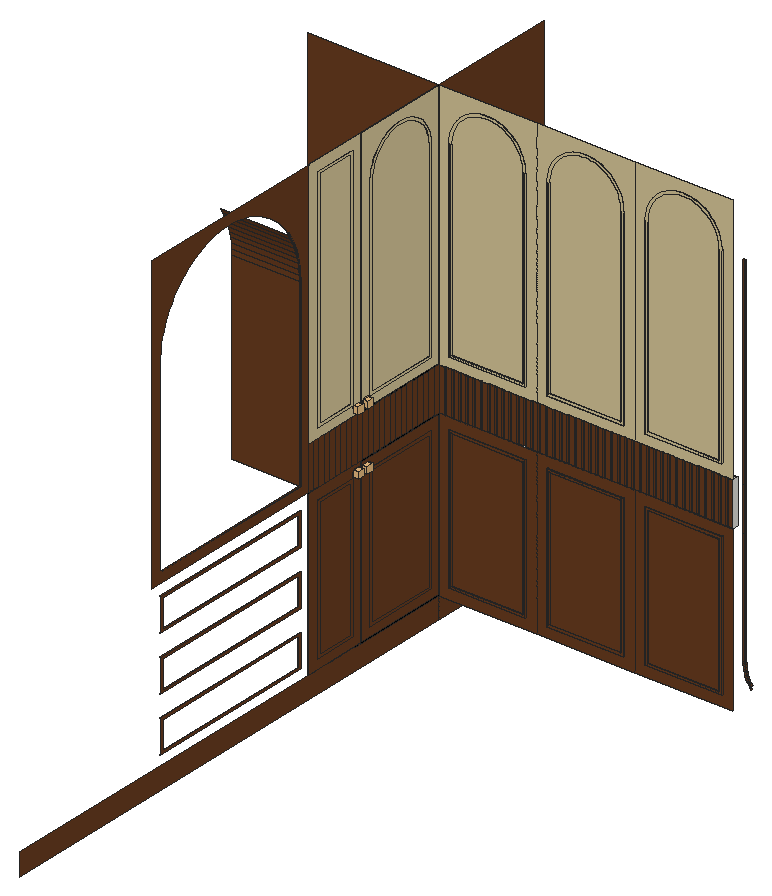
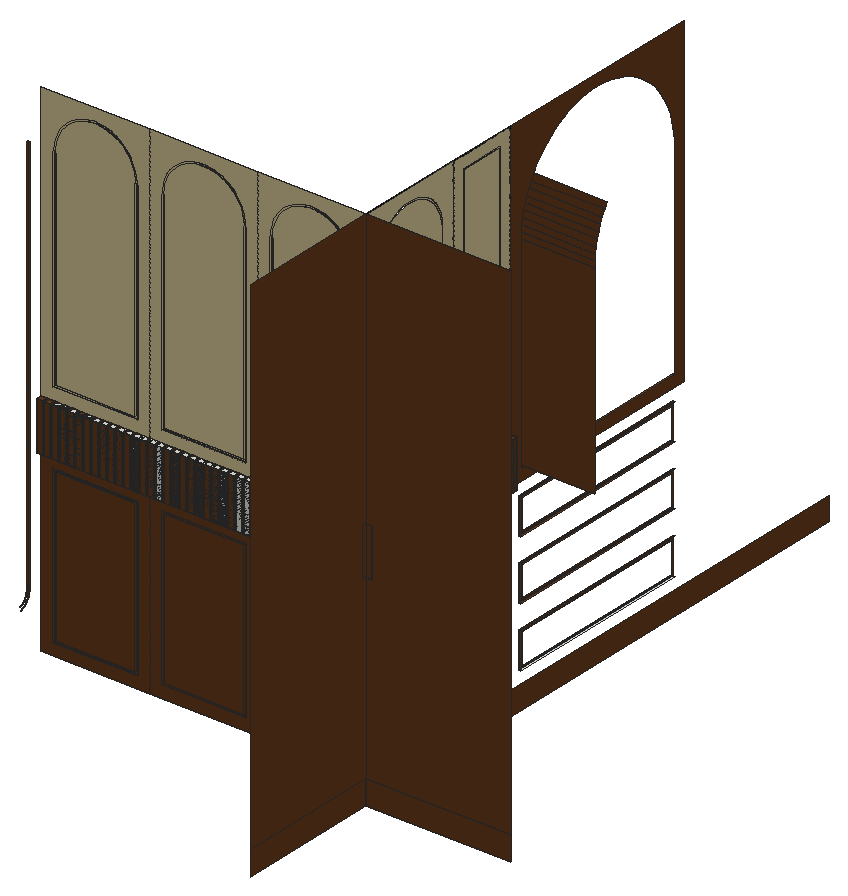
# SketchUp Ruby script. Lengths in inches.
U = 1.inch
M = Sketchup.active_model
def pt(a) = Geom::Point3d.new(a.map { |v| v * U })
def face(e, loops, mat)
  f = e.add_face(loops[0].map { |a| pt(a) })
  loops[1..].each { |l| e.add_face(l.map { |a| pt(a) }).erase! }
  f.material = f.back_material = mat if mat
  f
end
# faces: each face lists its corners as indices into pts; further lists are holes
def faces(e, pts, list, mat = nil) = list.each { |f| face(e, (f[0].is_a?(Array) ? f : [f]).map { |l| l.map { |i| pts[i] } }, mat) }
# xy, xz, yz: faces in a plane at the given z, y or x. An outline is a flat list of corners, or four numbers for a rectangle; further outlines are holes
def ring(l) = l.size == 4 ? [[l[0], l[1]], [l[2], l[1]], [l[2], l[3]], [l[0], l[3]]] : l.each_slice(2).to_a
def flat(e, list, mat, &to3) = list.each { |f| face(e, (f[0].is_a?(Array) ? f : [f]).map { |l| ring(l).map { |u, v| to3.(u, v) } }, mat) }
def xy(e, z, list, mat = nil) = flat(e, list, mat) { |x, y| [x, y, z] }
def xz(e, y, list, mat = nil) = flat(e, list, mat) { |x, z| [x, y, z] }
def yz(e, x, list, mat = nil) = flat(e, list, mat) { |y, z| [x, y, z] }
def lines(e, pts, list) = list.each { |a, b| e.add_line(pt(pts[a]), pt(pts[b])) }
# prism: a flat outline (further loops are holes) pulled along v
def prism(e, loops, v, mat = nil)
  f = face(e, loops, mat); d = Geom::Vector3d.new(v.map { |x| x * U })
  f.pushpull(f.normal.samedirection?(d) ? d.length : -d.length)
end
def box(e, o, s, mat = nil) = prism(e, [[o, [o[0] + s[0], o[1], o[2]], [o[0] + s[0], o[1] + s[1], o[2]], [o[0], o[1] + s[1], o[2]]]], [0, 0, s[2]], mat)
def at(x, y, z, deg = 0) = Geom::Transformation.translation(pt([x, y, z])) * Geom::Transformation.rotation(ORIGIN, Z_AXIS, deg.degrees)
def axes(o, x, y, z) = Geom::Transformation.new([*x, 0, *y, 0, *z, 0, *pt(o).to_a, 1])
def part(name) = M.definitions.add(name)
# library, detail: a bought-in or finely detailed component or shape, given as its bounding box
def library(name, o, s) = part(name).tap { |d| box(d.entities, o, s) }
def detail(e, o, s) = box(e.add_group.entities, o, s)
def put(e, d, t, mat = nil) = e.add_instance(d, t).tap { |i| i.material = mat if mat }
def group(e, t, mat = nil) = e.add_group.tap { |g| g.transformation = t; g.material = mat if mat }.entities
root = M.entities
M.materials.add("138_plaster painted wall texture-seamless").color = [214, 198, 153]
M.materials.add("[0137_Black]").color = [0, 0, 0]
M.materials.add("[Wood Veneer 01]").color = [104, 60, 32]
c1 = part("Group\#7")
box(c1.entities,[0,0,0],[1,1,8])
c2 = library("Group\#17",[0,0,0],[1.625,1.625,1.31])
c3 = part("Square post")
box(c3.entities,[0,0,0],[1,1,8])
xy(root,6,[[24,56,24.2,88],[24,92,24.2,100],[24,104,24.2,118],[26,119.8,40,120],[44,119.8,58,120]])
xy(root,6,[[62,119.8,76,120]],"[Wood Veneer 01]")
xy(root,6.4,[[24,56.4,24.2,87.6],[24,92.4,24.2,99.6],[24,104.4,24.2,117.6],[26.4,119.8,39.6,120],[44.4,119.8,57.6,120],
  [62.4,119.8,75.6,120]],"[Wood Veneer 01]")
xy(root,11.6,[[24,56.4,24.2,87.6]])
xy(root,12,[[24,56,24.2,88]],"[Wood Veneer 01]")
xy(root,16,[[24,56,24.2,88]],"[Wood Veneer 01]")
xy(root,16.4,[[24,56.4,24.2,87.6]],"[Wood Veneer 01]")
xy(root,21.6,[[24,56.4,24.2,87.6]],"[Wood Veneer 01]")
xy(root,22,[[24,56,24.2,88]],"[Wood Veneer 01]")
xy(root,26,[[24,56,24.2,88]],"[Wood Veneer 01]")
xy(root,26.4,[[24,56.4,24.2,87.6]],"[Wood Veneer 01]")
xy(root,31.6,[[24,56.4,24.2,87.6],[24,92.4,24.2,99.6],[24,104.4,24.2,117.6],[26.4,119.8,39.6,120],[44.4,119.8,57.6,120],
  [62.4,119.8,75.6,120]],"[Wood Veneer 01]")
xy(root,32,[[24,56,24.2,88],[24,92,24.2,100],[24,104,24.2,118],[26,119.8,40,120],[44,119.8,58,120],
  [62,119.8,76,120]],"[Wood Veneer 01]")
xy(root,34,[[24,120,42,121],[42,120,60,121],[60,120,78,121]])
xy(root,34,[[23,90,24,102],[23,102,24,120]],"[Wood Veneer 01]")
xy(root,36,[[24,56,24.2,88]],"[Wood Veneer 01]")
xy(root,42,[[24,120,42,121],[42,120,60,121],[60,120,78,121]])
xy(root,42,[[23,90,24,102],[23,102,24,120]],"[Wood Veneer 01]")
xy(root,44,[[24,92,24.2,100],[24,104,24.2,118],[26,119.8,40,120],[44,119.8,58,120],[62,119.8,76,120]])
xy(root,44.4,[[24,92.4,24.2,99.6],[24,104.4,24.2,117.6]])
xy(root,44.4,[[26.4,119.8,39.6,120],[44.4,119.8,57.6,120],[62.4,119.8,75.6,120]],"138_plaster painted wall texture-seamless")
xz(root,87.6,[[24,6.4,24.2,11.6],[24,16.4,24.2,21.6],[24,26.4,24.2,31.6],[12,36.4,24.2,70]],"[Wood Veneer 01]")
xz(root,88,[[24,6,24.2,12],[24,16,24.2,22],[24,26,24.2,32],[24,36,24.2,42],[24,42,24.2,70]],"[Wood Veneer 01]")
xz(root,90,[[23,34,24,42]])
xz(root,92,[[24,44,24.2,86]])
xz(root,92,[[24,6,24.2,32]],"[Wood Veneer 01]")
xz(root,92.4,[[24,44.4,24.2,85.6]])
xz(root,92.4,[[24,6.4,24.2,31.6]],"[Wood Veneer 01]")
xz(root,99.6,[[24,44.4,24.2,85.6]])
xz(root,99.6,[[24,6.4,24.2,31.6]],"[Wood Veneer 01]")
xz(root,100,[[24,44,24.2,86]])
xz(root,100,[[24,6,24.2,32]],"[Wood Veneer 01]")
xz(root,104,[[24,44,24.2,79]])
xz(root,104,[[24,6,24.2,32]],"[Wood Veneer 01]")
xz(root,104.4,[[24,44.4,24.2,79]])
xz(root,104.4,[[24,6.4,24.2,31.6]],"[Wood Veneer 01]")
xz(root,117.6,[[24,44.4,24.2,79]])
xz(root,117.6,[[24,6.4,24.2,31.6]],"[Wood Veneer 01]")
xz(root,118,[[24,44,24.2,79]])
xz(root,118,[[24,6,24.2,32]],"[Wood Veneer 01]")
xz(root,119.8,[[[26,44,40,44,40,79,39.99,79.46,39.94,79.91,39.87,80.37,39.76,80.8125,39.63,81.25,39.47,81.68,39.28,82.1,39.0625,82.5,38.82,82.89,38.55,83.26,38.26,83.62,37.95,83.95,37.62,84.26,37.26,84.55,36.89,84.82,36.5,85.0625,36.1,85.28,35.68,85.47,35.25,85.63,34.8125,85.76,34.37,85.87,33.91,85.94,33.46,85.99,33,86,32.54,85.99,32.09,85.94,31.63,85.87,31.1875,85.76,30.75,85.63,30.32,85.47,29.9,85.28,29.5,85.0625,29.11,84.82,28.74,84.55,28.38,84.26,28.05,83.95,27.74,83.62,27.45,83.26,27.18,82.89,26.9375,82.5,26.72,82.1,26.53,81.68,26.37,81.25,26.24,80.8125,26.13,80.37,26.06,79.91,26.01,79.46,26,79],[26.4,44.4,26.4,79,26.41,79.43,26.46,79.86,26.53,80.29,26.625,80.71,26.75,81.12,26.9,81.53,27.08,81.92,27.28,82.3,27.51,82.67,27.76,83.02,28.04,83.35,28.33,83.67,28.65,83.96,28.98,84.24,29.33,84.49,29.7,84.72,30.08,84.92,30.47,85.1,30.88,85.25,31.29,85.375,31.71,85.47,32.14,85.54,32.57,85.59,33,85.6,33.43,85.59,33.86,85.54,34.29,85.47,34.71,85.375,35.12,85.25,35.53,85.1,35.92,84.92,36.3,84.72,36.67,84.49,37.02,84.24,37.35,83.96,37.67,83.67,37.96,83.35,38.24,83.02,38.49,82.67,38.72,82.3,38.92,81.92,39.1,81.53,39.25,81.12,39.375,80.71,39.47,80.29,39.54,79.86,39.59,79.43,39.6,79,39.6,44.4]],[[44,44,58,44,58,79,57.99,79.46,57.94,79.91,57.87,80.37,57.76,80.8125,57.63,81.25,57.47,81.68,57.28,82.1,57.0625,82.5,56.82,82.89,56.55,83.26,56.26,83.62,55.95,83.95,55.62,84.26,55.26,84.55,54.89,84.82,54.5,85.0625,54.1,85.28,53.68,85.47,53.25,85.63,52.8125,85.76,52.37,85.87,51.91,85.94,51.46,85.99,51,86,50.54,85.99,50.09,85.94,49.63,85.87,49.1875,85.76,48.75,85.63,48.32,85.47,47.9,85.28,47.5,85.0625,47.11,84.82,46.74,84.55,46.38,84.26,46.05,83.95,45.74,83.62,45.45,83.26,45.18,82.89,44.9375,82.5,44.72,82.1,44.53,81.68,44.37,81.25,44.24,80.8125,44.13,80.37,44.06,79.91,44.01,79.46,44,79],[44.4,44.4,44.4,79,44.41,79.43,44.46,79.86,44.53,80.29,44.625,80.71,44.75,81.12,44.9,81.53,45.08,81.92,45.28,82.3,45.51,82.67,45.76,83.02,46.04,83.35,46.33,83.67,46.65,83.96,46.98,84.24,47.33,84.49,47.7,84.72,48.08,84.92,48.47,85.1,48.88,85.25,49.29,85.375,49.71,85.47,50.14,85.54,50.57,85.59,51,85.6,51.43,85.59,51.86,85.54,52.29,85.47,52.71,85.375,53.12,85.25,53.53,85.1,53.92,84.92,54.3,84.72,54.67,84.49,55.02,84.24,55.35,83.96,55.67,83.67,55.96,83.35,56.24,83.02,56.49,82.67,56.72,82.3,56.92,81.92,57.1,81.53,57.25,81.12,57.375,80.71,57.47,80.29,57.54,79.86,57.59,79.43,57.6,79,57.6,44.4]],[[62,44,76,44,76,79,75.99,79.46,75.94,79.91,75.87,80.37,75.76,80.8125,75.63,81.25,75.47,81.68,75.28,82.1,75.0625,82.5,74.82,82.89,74.55,83.26,74.26,83.62,73.95,83.95,73.62,84.26,73.26,84.55,72.89,84.82,72.5,85.0625,72.1,85.28,71.68,85.47,71.25,85.63,70.8125,85.76,70.37,85.87,69.91,85.94,69.46,85.99,69,86,68.54,85.99,68.09,85.94,67.63,85.87,67.1875,85.76,66.75,85.63,66.32,85.47,65.9,85.28,65.5,85.0625,65.11,84.82,64.74,84.55,64.38,84.26,64.05,83.95,63.74,83.62,63.45,83.26,63.18,82.89,62.9375,82.5,62.72,82.1,62.53,81.68,62.37,81.25,62.24,80.8125,62.13,80.37,62.06,79.91,62.01,79.46,62,79],[62.4,44.4,62.4,79,62.41,79.43,62.46,79.86,62.53,80.29,62.625,80.71,62.75,81.12,62.9,81.53,63.08,81.92,63.28,82.3,63.51,82.67,63.76,83.02,64.04,83.35,64.33,83.67,64.65,83.96,64.98,84.24,65.33,84.49,65.7,84.72,66.08,84.92,66.47,85.1,66.88,85.25,67.29,85.375,67.71,85.47,68.14,85.54,68.57,85.59,69,85.6,69.43,85.59,69.86,85.54,70.29,85.47,70.71,85.375,71.12,85.25,71.53,85.1,71.92,84.92,72.3,84.72,72.67,84.49,73.02,84.24,73.35,83.96,73.67,83.67,73.96,83.35,74.24,83.02,74.49,82.67,74.72,82.3,74.92,81.92,75.1,81.53,75.25,81.12,75.375,80.71,75.47,80.29,75.54,79.86,75.59,79.43,75.6,79,75.6,44.4]]],"138_plaster painted wall texture-seamless")
xz(root,119.8,[[[26,6,40,32],[26.4,6.4,39.6,31.6]],[[44,6,58,32],[44.4,6.4,57.6,31.6]],[[62,6,76,32],[62.4,6.4,75.6,31.6]]],"[Wood Veneer 01]")
xz(root,120,[[[24,42,42,88],[26,44,26,79,26.01,79.46,26.06,79.91,26.13,80.37,26.24,80.8125,26.37,81.25,26.53,81.68,26.72,82.1,26.9375,82.5,27.18,82.89,27.45,83.26,27.74,83.62,28.05,83.95,28.38,84.26,28.74,84.55,29.11,84.82,29.5,85.0625,29.9,85.28,30.32,85.47,30.75,85.63,31.1875,85.76,31.63,85.87,32.09,85.94,32.54,85.99,33,86,33.46,85.99,33.91,85.94,34.37,85.87,34.8125,85.76,35.25,85.63,35.68,85.47,36.1,85.28,36.5,85.0625,36.89,84.82,37.26,84.55,37.62,84.26,37.95,83.95,38.26,83.62,38.55,83.26,38.82,82.89,39.0625,82.5,39.28,82.1,39.47,81.68,39.63,81.25,39.76,80.8125,39.87,80.37,39.94,79.91,39.99,79.46,40,79,40,44]],[[42,42,60,88],[44,44,44,79,44.01,79.46,44.06,79.91,44.13,80.37,44.24,80.8125,44.37,81.25,44.53,81.68,44.72,82.1,44.9375,82.5,45.18,82.89,45.45,83.26,45.74,83.62,46.05,83.95,46.38,84.26,46.74,84.55,47.11,84.82,47.5,85.0625,47.9,85.28,48.32,85.47,48.75,85.63,49.1875,85.76,49.63,85.87,50.09,85.94,50.54,85.99,51,86,51.46,85.99,51.91,85.94,52.37,85.87,52.8125,85.76,53.25,85.63,53.68,85.47,54.1,85.28,54.5,85.0625,54.89,84.82,55.26,84.55,55.62,84.26,55.95,83.95,56.26,83.62,56.55,83.26,56.82,82.89,57.0625,82.5,57.28,82.1,57.47,81.68,57.63,81.25,57.76,80.8125,57.87,80.37,57.94,79.91,57.99,79.46,58,79,58,44]],[[60,42,78,88],[62,44,62,79,62.01,79.46,62.06,79.91,62.13,80.37,62.24,80.8125,62.37,81.25,62.53,81.68,62.72,82.1,62.9375,82.5,63.18,82.89,63.45,83.26,63.74,83.62,64.05,83.95,64.38,84.26,64.74,84.55,65.11,84.82,65.5,85.0625,65.9,85.28,66.32,85.47,66.75,85.63,67.1875,85.76,67.63,85.87,68.09,85.94,68.54,85.99,69,86,69.46,85.99,69.91,85.94,70.37,85.87,70.8125,85.76,71.25,85.63,71.68,85.47,72.1,85.28,72.5,85.0625,72.89,84.82,73.26,84.55,73.62,84.26,73.95,83.95,74.26,83.62,74.55,83.26,74.82,82.89,75.0625,82.5,75.28,82.1,75.47,81.68,75.63,81.25,75.76,80.8125,75.87,80.37,75.94,79.91,75.99,79.46,76,79,76,44]],[26.4,44.4,39.6,44.4,39.6,79,39.59,79.43,39.54,79.86,39.47,80.29,39.375,80.71,39.25,81.12,39.1,81.53,38.92,81.92,38.72,82.3,38.49,82.67,38.24,83.02,37.96,83.35,37.67,83.67,37.35,83.96,37.02,84.24,36.67,84.49,36.3,84.72,35.92,84.92,35.53,85.1,35.12,85.25,34.71,85.375,34.29,85.47,33.86,85.54,33.43,85.59,33,85.6,32.57,85.59,32.14,85.54,31.71,85.47,31.29,85.375,30.88,85.25,30.47,85.1,30.08,84.92,29.7,84.72,29.33,84.49,28.98,84.24,28.65,83.96,28.33,83.67,28.04,83.35,27.76,83.02,27.51,82.67,27.28,82.3,27.08,81.92,26.9,81.53,26.75,81.12,26.625,80.71,26.53,80.29,26.46,79.86,26.41,79.43,26.4,79],[44.4,44.4,57.6,44.4,57.6,79,57.59,79.43,57.54,79.86,57.47,80.29,57.375,80.71,57.25,81.12,57.1,81.53,56.92,81.92,56.72,82.3,56.49,82.67,56.24,83.02,55.96,83.35,55.67,83.67,55.35,83.96,55.02,84.24,54.67,84.49,54.3,84.72,53.92,84.92,53.53,85.1,53.12,85.25,52.71,85.375,52.29,85.47,51.86,85.54,51.43,85.59,51,85.6,50.57,85.59,50.14,85.54,49.71,85.47,49.29,85.375,48.88,85.25,48.47,85.1,48.08,84.92,47.7,84.72,47.33,84.49,46.98,84.24,46.65,83.96,46.33,83.67,46.04,83.35,45.76,83.02,45.51,82.67,45.28,82.3,45.08,81.92,44.9,81.53,44.75,81.12,44.625,80.71,44.53,80.29,44.46,79.86,44.41,79.43,44.4,79],
  [62.4,44.4,75.6,44.4,75.6,79,75.59,79.43,75.54,79.86,75.47,80.29,75.375,80.71,75.25,81.12,75.1,81.53,74.92,81.92,74.72,82.3,74.49,82.67,74.24,83.02,73.96,83.35,73.67,83.67,73.35,83.96,73.02,84.24,72.67,84.49,72.3,84.72,71.92,84.92,71.53,85.1,71.12,85.25,70.71,85.375,70.29,85.47,69.86,85.54,69.43,85.59,69,85.6,68.57,85.59,68.14,85.54,67.71,85.47,67.29,85.375,66.88,85.25,66.47,85.1,66.08,84.92,65.7,84.72,65.33,84.49,64.98,84.24,64.65,83.96,64.33,83.67,64.04,83.35,63.76,83.02,63.51,82.67,63.28,82.3,63.08,81.92,62.9,81.53,62.75,81.12,62.625,80.71,62.53,80.29,62.46,79.86,62.41,79.43,62.4,79]],"138_plaster painted wall texture-seamless")
xz(root,120,[[0,0,24,4],[0,4,0,88,24,88,24,42,23,42,23,34,24,34,24,4],[[24,4,42,34],[26,6,40,32]],[[42,4,60,34],[44,6,58,32]],[[60,4,78,34],[62,6,76,32]],
  [26.4,6.4,39.6,31.6],[44.4,6.4,57.6,31.6],[62.4,6.4,75.6,31.6]],"[Wood Veneer 01]")
xz(root,121,[[24,34,78,42]])
yz(root,23,[[90,34,120,42]],"[Wood Veneer 01]")
yz(root,24,[[[90.1,42.1,101.9,87.9],[92,44,100,86]],[[102.1,42.1,119.9,87.9],[104,44,104,79,104.01,79.46,104.06,79.91,104.13,80.37,104.24,80.8125,104.37,81.25,104.53,81.68,104.72,82.1,104.9375,82.5,105.18,82.89,105.45,83.26,105.74,83.62,106.05,83.95,106.38,84.26,106.74,84.55,107.11,84.82,107.5,85.0625,107.9,85.28,108.32,85.47,108.75,85.63,109.1875,85.76,109.63,85.87,110.09,85.94,110.54,85.99,111,86,111.46,85.99,111.91,85.94,112.37,85.87,112.8125,85.76,113.25,85.63,113.68,85.47,114.1,85.28,114.5,85.0625,114.89,84.82,115.26,84.55,115.62,84.26,115.95,83.95,116.26,83.62,116.55,83.26,116.82,82.89,117.0625,82.5,117.28,82.1,117.47,81.68,117.63,81.25,117.76,80.8125,117.87,80.37,117.94,79.91,117.99,79.46,118,79,118,44]],[92.4,44.4,99.6,85.6],[104.4,44.4,117.6,44.4,117.6,79,117.59,79.43,117.54,79.86,117.47,80.29,117.375,80.71,117.25,81.12,117.1,81.53,116.92,81.92,116.72,82.3,116.49,82.67,116.24,83.02,115.96,83.35,115.67,83.67,115.35,83.96,115.02,84.24,114.67,84.49,114.3,84.72,113.92,84.92,113.53,85.1,113.12,85.25,112.71,85.375,112.29,85.47,111.86,85.54,111.43,85.59,111,85.6,110.57,85.59,110.14,85.54,109.71,85.47,109.29,85.375,108.88,85.25,108.47,85.1,108.08,84.92,107.7,84.72,107.33,84.49,106.98,84.24,106.65,83.96,106.33,83.67,106.04,83.35,105.76,83.02,105.51,82.67,105.28,82.3,105.08,81.92,104.9,81.53,104.75,81.12,104.625,80.71,104.53,80.29,104.46,79.86,104.41,79.43,104.4,79]],"138_plaster painted wall texture-seamless")
yz(root,24,[[[90,4,102,34],[90.1,4.1,101.9,33.9]],[[102,4,120,34],[102.1,4.1,119.9,33.9]],[[90,42,102,88],[90.1,42.1,101.9,87.9]],[[102,42,120,88],[102.1,42.1,119.9,87.9]]],"[0137_Black]")
yz(root,24,[[24,0,120,4],[120,0,144,4],[120,4,120,34,121,34,121,42,120,42,120,88,144,88,144,4],[[90.1,4.1,101.9,33.9],[92,6,100,32]],[[102.1,4.1,119.9,33.9],[104,6,118,32]],
  [92.4,6.4,99.6,31.6],[104.4,6.4,117.6,31.6],[[54.1,34.1,89.9,87.9],[56,36,56,70,56.03,71.05,56.14,72.09,56.31,73.12,56.55,74.14,56.85,75.14,57.22,76.12,57.65,77.08,58.14,78,58.7,78.89,59.31,79.74,59.97,80.55,60.6875,81.3125,61.45,82.03,62.26,82.69,63.11,83.3,64,83.86,64.92,84.35,65.88,84.78,66.86,85.15,67.86,85.45,68.88,85.69,69.91,85.86,70.95,85.97,72,86,73.05,85.97,74.09,85.86,75.12,85.69,76.14,85.45,77.14,85.15,78.12,84.78,79.08,84.35,80,83.86,80.89,83.3,81.74,82.69,82.55,82.03,83.3125,81.3125,84.03,80.55,84.69,79.74,85.3,78.89,85.86,78,86.35,77.08,86.78,76.12,87.15,75.14,87.45,74.14,87.69,73.12,87.86,72.09,87.97,71.05,88,70,88,36]]],"[Wood Veneer 01]")
yz(root,24.2,[[[92,44,100,86],[92.4,44.4,99.6,85.6]],[[104,44,118,44,118,79,117.99,79.46,117.94,79.91,117.87,80.37,117.76,80.8125,117.63,81.25,117.47,81.68,117.28,82.1,117.0625,82.5,116.82,82.89,116.55,83.26,116.26,83.62,115.95,83.95,115.62,84.26,115.26,84.55,114.89,84.82,114.5,85.0625,114.1,85.28,113.68,85.47,113.25,85.63,112.8125,85.76,112.37,85.87,111.91,85.94,111.46,85.99,111,86,110.54,85.99,110.09,85.94,109.63,85.87,109.1875,85.76,108.75,85.63,108.32,85.47,107.9,85.28,107.5,85.0625,107.11,84.82,106.74,84.55,106.38,84.26,106.05,83.95,105.74,83.62,105.45,83.26,105.18,82.89,104.9375,82.5,104.72,82.1,104.53,81.68,104.37,81.25,104.24,80.8125,104.13,80.37,104.06,79.91,104.01,79.46,104,79],[104.4,44.4,104.4,79,104.41,79.43,104.46,79.86,104.53,80.29,104.625,80.71,104.75,81.12,104.9,81.53,105.08,81.92,105.28,82.3,105.51,82.67,105.76,83.02,106.04,83.35,106.33,83.67,106.65,83.96,106.98,84.24,107.33,84.49,107.7,84.72,108.08,84.92,108.47,85.1,108.88,85.25,109.29,85.375,109.71,85.47,110.14,85.54,110.57,85.59,111,85.6,111.43,85.59,111.86,85.54,112.29,85.47,112.71,85.375,113.12,85.25,113.53,85.1,113.92,84.92,114.3,84.72,114.67,84.49,115.02,84.24,115.35,83.96,115.67,83.67,115.96,83.35,116.24,83.02,116.49,82.67,116.72,82.3,116.92,81.92,117.1,81.53,117.25,81.12,117.375,80.71,117.47,80.29,117.54,79.86,117.59,79.43,117.6,79,117.6,44.4]]],"138_plaster painted wall texture-seamless")
yz(root,24.2,[[[56,6,88,12],[56.4,6.4,87.6,11.6]],[[92,6,100,32],[92.4,6.4,99.6,31.6]],[[104,6,118,32],[104.4,6.4,117.6,31.6]],[[56,16,88,22],[56.4,16.4,87.6,21.6]],[[56,26,88,32],[56.4,26.4,87.6,31.6]]],"[Wood Veneer 01]")
yz(root,26,[[119.8,44,120,79]])
yz(root,26,[[119.8,6,120,32]],"[Wood Veneer 01]")
yz(root,26.4,[[119.8,44.4,120,79]],"138_plaster painted wall texture-seamless")
yz(root,26.4,[[119.8,6.4,120,31.6]],"[Wood Veneer 01]")
yz(root,39.6,[[119.8,44.4,120,79]])
yz(root,39.6,[[119.8,6.4,120,31.6]],"[Wood Veneer 01]")
yz(root,40,[[119.8,44,120,79]],"138_plaster painted wall texture-seamless")
yz(root,40,[[119.8,6,120,32]],"[Wood Veneer 01]")
yz(root,44,[[119.8,44,120,79]])
yz(root,44,[[119.8,6,120,32]],"[Wood Veneer 01]")
yz(root,44.4,[[119.8,44.4,120,79]],"138_plaster painted wall texture-seamless")
yz(root,44.4,[[119.8,6.4,120,31.6]],"[Wood Veneer 01]")
yz(root,57.6,[[119.8,44.4,120,79]])
yz(root,57.6,[[119.8,6.4,120,31.6]],"[Wood Veneer 01]")
yz(root,58,[[119.8,44,120,79]],"138_plaster painted wall texture-seamless")
yz(root,58,[[119.8,6,120,32]],"[Wood Veneer 01]")
yz(root,62,[[119.8,44,120,79]])
yz(root,62,[[119.8,6,120,32]],"[Wood Veneer 01]")
yz(root,62.4,[[119.8,44.4,120,79]],"138_plaster painted wall texture-seamless")
yz(root,62.4,[[119.8,6.4,120,31.6]],"[Wood Veneer 01]")
yz(root,75.6,[[119.8,44.4,120,79]])
yz(root,75.6,[[119.8,6.4,120,31.6]],"[Wood Veneer 01]")
yz(root,76,[[119.8,44,120,79]],"138_plaster painted wall texture-seamless")
yz(root,76,[[119.8,6,120,32]],"[Wood Veneer 01]")
yz(root,78,[[120,34,121,42]])
yz(root,80,[[119.8,13,120,34],[119.8,34,120,42],[119.8,42,120,79]],"[Wood Veneer 01]")
yz(root,80.4,[[119.8,13,120,34],[119.8,34,120,42],[119.8,42,120,79]],"[Wood Veneer 01]")
p = [[81.18,120,9.11],[81.45,120,8.74],[81.45,119.8,8.74],[81.18,119.8,9.11],[80.9375,120,9.5],[80.9375,119.8,9.5],
  [81.51,120,9.33],[81.28,120,9.7],[81.28,119.8,9.7],[81.51,119.8,9.33],[80.72,120,9.9],[80.72,119.8,9.9],
  [81.08,120,10.08],[81.08,119.8,10.08],[80.53,120,10.32],[80.53,119.8,10.32],[80.9,120,10.47],[80.9,119.8,10.47],
  [80.37,120,10.75],[80.37,119.8,10.75],[80.75,120,10.88],[80.75,119.8,10.88],[80.24,120,11.1875],[80.24,119.8,11.1875],
  [80.625,120,11.29],[80.625,119.8,11.29],[80.13,120,11.63],[80.13,119.8,11.63],[80.53,120,11.71],[80.53,119.8,11.71],
  [80.06,120,12.09],[80.06,119.8,12.09],[80.46,120,12.14],[80.46,119.8,12.14],[80.01,120,12.54],[80.01,119.8,12.54],
  [80.41,120,12.57],[80.41,119.8,12.57],[80,120,13],[80,119.8,13],[80.4,120,13],[80.4,119.8,13],
  [12,87.6,70],[24.2,87.6,70],[24.2,87.57,71.02],[12,87.57,71.02],[24,88,70],[24,87.97,71.05],
  [24.2,87.97,71.05],[24.2,88,70],[24.2,87.47,72.04],[12,87.47,72.04],[24,87.86,72.09],[24.2,87.86,72.09],
  [24.2,87.3,73.04],[12,87.3,73.04],[24,87.69,73.12],[24.2,87.69,73.12],[24.2,87.07,74.04],[12,87.07,74.04],
  [24,87.45,74.14],[24.2,87.45,74.14],[24.2,86.77,75.01],[12,86.77,75.01],[24,87.15,75.14],[24.2,87.15,75.14],
  [24.2,86.41,75.97],[12,86.41,75.97],[24,86.78,76.12],[24.2,86.78,76.12],[24.2,85.99,76.9],[12,85.99,76.9],
  [24,86.35,77.08],[24.2,86.35,77.08],[24.2,85.51,77.8],[12,85.51,77.8],[24,85.86,78],[24.2,85.86,78],
  [24.2,84.97,78.67],[12,84.97,78.67],[24,85.3,78.89],[24.2,85.3,78.89]]
faces(root,p,[[0,1,2,3],[4,0,3,5],[6,7,8,9],[10,4,5,11],[7,12,13,8],[14,10,11,15],[12,16,17,13],[18,14,15,19],
  [16,20,21,17],[22,18,19,23],[20,24,25,21],[26,22,23,27],[24,28,29,25],[30,26,27,31],[28,32,33,29],[34,30,31,35],
  [32,36,37,33],[38,34,35,39],[36,40,41,37],[42,43,44,45],[46,47,48,49],[45,44,50,51],[47,52,53,48],[51,50,54,55],
  [52,56,57,53],[55,54,58,59],[56,60,61,57],[59,58,62,63],[60,64,65,61],[63,62,66,67],[64,68,69,65],[67,66,70,71],
  [68,72,73,69],[71,70,74,75],[72,76,77,73],[75,74,78,79],[76,80,81,77]],"[Wood Veneer 01]")
put(root,c1,at(23,90,34),"[Wood Veneer 01]")
put(root,c1,at(23,91.26,34),"[Wood Veneer 01]")
put(root,c1,at(23,92.52,34),"[Wood Veneer 01]")
put(root,c1,at(23,93.78,34),"[Wood Veneer 01]")
put(root,c1,at(23,95.04,34),"[Wood Veneer 01]")
put(root,c1,at(23,96.3,34),"[Wood Veneer 01]")
put(root,c1,at(23,97.57,34),"[Wood Veneer 01]")
put(root,c1,at(23,98.83,34),"[Wood Veneer 01]")
put(root,c1,at(23,100.09,34),"[Wood Veneer 01]")
put(root,c2,axes([24,101.5,43.94],[0,-0.74,0],[0,0,-0.74],[0.74,0,0]),"[Wood Veneer 01]")
put(root,c2,axes([24,101.57,33.29],[0,-0.74,0],[0,0,-0.74],[0.74,0,0]),"[Wood Veneer 01]")
put(root,c1,at(23,101.35,34),"[Wood Veneer 01]")
put(root,c2,axes([24,103.57,33.29],[0,-0.74,0],[0,0,-0.74],[0.74,0,0]),"[Wood Veneer 01]")
put(root,c2,axes([24,103.6875,43.94],[0,-0.74,0],[0,0,-0.74],[0.74,0,0]),"[Wood Veneer 01]")
put(root,c1,at(23,102.61,34),"[Wood Veneer 01]")
put(root,c1,at(23,103.87,34),"[Wood Veneer 01]")
put(root,c1,at(23,105.13,34),"[Wood Veneer 01]")
put(root,c1,at(23,106.39,34),"[Wood Veneer 01]")
put(root,c1,at(23,107.65,34),"[Wood Veneer 01]")
put(root,c1,at(23,108.91,34),"[Wood Veneer 01]")
put(root,c1,at(23,110.17,34),"[Wood Veneer 01]")
put(root,c1,at(23,111.43,34),"[Wood Veneer 01]")
put(root,c1,at(23,112.7,34),"[Wood Veneer 01]")
put(root,c1,at(23,113.96,34),"[Wood Veneer 01]")
put(root,c1,at(23,115.22,34),"[Wood Veneer 01]")
put(root,c1,at(23,116.48,34),"[Wood Veneer 01]")
put(root,c1,at(23,117.74,34),"[Wood Veneer 01]")
put(root,c1,at(23,119,34),"[Wood Veneer 01]")
g1 = group(root,at(24,120,34),"[Wood Veneer 01]")
put(g1,c3,at(0,0,0))
put(g1,c3,at(29.15,0,0))
put(g1,c3,at(45.05,0,0))
put(g1,c3,at(41.08,0,0))
put(g1,c3,at(17.22,0,0))
put(g1,c3,at(27.82,0,0))
put(g1,c3,at(43.73,0,0))
put(g1,c3,at(11.92,0,0))
put(g1,c3,at(34.45,0,0))
put(g1,c3,at(3.98,0,0))
put(g1,c3,at(6.625,0,0))
put(g1,c3,at(39.75,0,0))
put(g1,c3,at(42.4,0,0))
put(g1,c3,at(49.03,0,0))
put(g1,c3,at(50.35,0,0))
put(g1,c3,at(46.375,0,0))
put(g1,c3,at(19.875,0,0))
put(g1,c3,at(18.55,0,0))
put(g1,c3,at(33.125,0,0))
put(g1,c3,at(38.43,0,0))
put(g1,c3,at(7.95,0,0))
put(g1,c3,at(51.68,0,0))
put(g1,c3,at(47.7,0,0))
put(g1,c3,at(53,0,0))
put(g1,c3,at(2.65,0,0))
put(g1,c3,at(13.25,0,0))
put(g1,c3,at(21.2,0,0))
put(g1,c3,at(31.8,0,0))
put(g1,c3,at(1.32,0,0))
put(g1,c3,at(14.58,0,0))
put(g1,c3,at(15.9,0,0))
put(g1,c3,at(37.1,0,0))
put(g1,c3,at(10.6,0,0))
put(g1,c3,at(5.3,0,0))
put(g1,c3,at(9.28,0,0))
put(g1,c3,at(22.52,0,0))
put(g1,c3,at(25.17,0,0))
put(g1,c3,at(26.5,0,0))
put(g1,c3,at(23.85,0,0))
put(g1,c3,at(35.78,0,0))
put(g1,c3,at(30.47,0,0))
